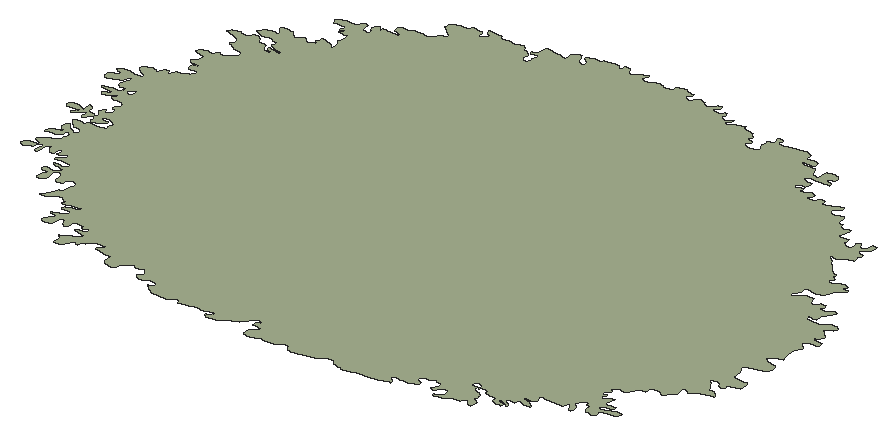
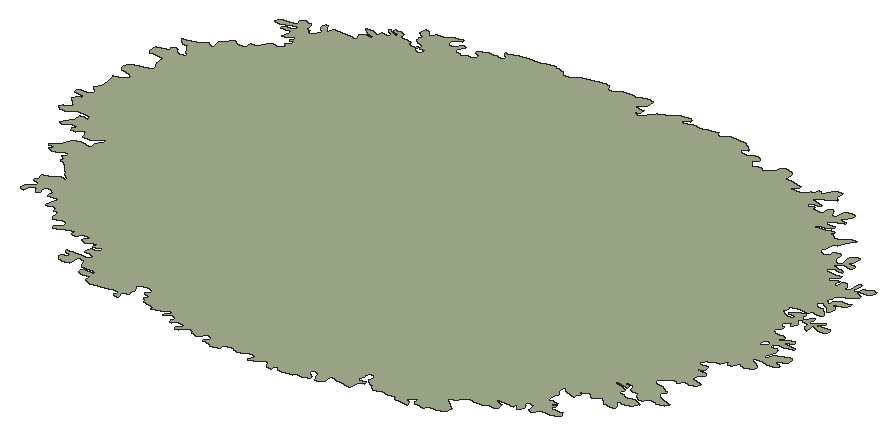
# SketchUp Ruby script. Lengths in inches.
U = 1.inch
M = Sketchup.active_model
def pt(a) = Geom::Point3d.new(a.map { |v| v * U })
def face(e, loops, mat)
  f = e.add_face(loops[0].map { |a| pt(a) })
  loops[1..].each { |l| e.add_face(l.map { |a| pt(a) }).erase! }
  f.material = f.back_material = mat if mat
  f
end
# faces: each face lists its corners as indices into pts; further lists are holes
def faces(e, pts, list, mat = nil) = list.each { |f| face(e, (f[0].is_a?(Array) ? f : [f]).map { |l| l.map { |i| pts[i] } }, mat) }
# xy, xz, yz: faces in a plane at the given z, y or x. An outline is a flat list of corners, or four numbers for a rectangle; further outlines are holes
def ring(l) = l.size == 4 ? [[l[0], l[1]], [l[2], l[1]], [l[2], l[3]], [l[0], l[3]]] : l.each_slice(2).to_a
def flat(e, list, mat, &to3) = list.each { |f| face(e, (f[0].is_a?(Array) ? f : [f]).map { |l| ring(l).map { |u, v| to3.(u, v) } }, mat) }
def xy(e, z, list, mat = nil) = flat(e, list, mat) { |x, y| [x, y, z] }
def xz(e, y, list, mat = nil) = flat(e, list, mat) { |x, z| [x, y, z] }
def yz(e, x, list, mat = nil) = flat(e, list, mat) { |y, z| [x, y, z] }
def lines(e, pts, list) = list.each { |a, b| e.add_line(pt(pts[a]), pt(pts[b])) }
# prism: a flat outline (further loops are holes) pulled along v
def prism(e, loops, v, mat = nil)
  f = face(e, loops, mat); d = Geom::Vector3d.new(v.map { |x| x * U })
  f.pushpull(f.normal.samedirection?(d) ? d.length : -d.length)
end
def box(e, o, s, mat = nil) = prism(e, [[o, [o[0] + s[0], o[1], o[2]], [o[0] + s[0], o[1] + s[1], o[2]], [o[0], o[1] + s[1], o[2]]]], [0, 0, s[2]], mat)
def at(x, y, z, deg = 0) = Geom::Transformation.translation(pt([x, y, z])) * Geom::Transformation.rotation(ORIGIN, Z_AXIS, deg.degrees)
def axes(o, x, y, z) = Geom::Transformation.new([*x, 0, *y, 0, *z, 0, *pt(o).to_a, 1])
def part(name) = M.definitions.add(name)
# library, detail: a bought-in or finely detailed component or shape, given as its bounding box
def library(name, o, s) = part(name).tap { |d| box(d.entities, o, s) }
def detail(e, o, s) = box(e.add_group.entities, o, s)
def put(e, d, t, mat = nil) = e.add_instance(d, t).tap { |i| i.material = mat if mat }
def group(e, t, mat = nil) = e.add_group.tap { |g| g.transformation = t; g.material = mat if mat }.entities
root = M.entities
M.materials.add("Boxwoodplan").color = [166, 177, 144]
xy(root,9.058,[[[182.292,67.129,182.181,67.133,182.086,67.159,182.03,67.215,182.028,67.317,182.054,67.382,182.118,67.445,182.167,67.509,182.225,67.606,182.039,67.635,181.949,67.644,181.969,67.732,182.055,67.79,182.086,67.8,182.081,67.846,181.992,67.877,181.876,67.837,181.779,67.706,181.636,67.551,181.475,67.464,181.37,67.441,181.309,67.416,181.293,67.373,181.149,67.281,180.955,67.251,180.866,67.26,180.786,67.306,180.786,67.328,180.831,67.359,180.922,67.437,180.99,67.483,180.901,67.498,180.788,67.48,180.668,67.436,180.572,67.445,180.475,67.454,180.378,67.447,180.251,67.403,180.051,67.356,179.962,67.349,179.924,67.443,179.916,67.465,179.849,67.473,179.76,67.454,179.591,67.336,179.391,67.328,179.161,67.353,178.994,67.446,178.853,67.61,179.036,67.702,178.936,67.756,178.8,67.772,178.674,67.749,178.602,67.697,178.521,67.672,178.405,67.738,178.363,67.806,178.451,67.847,178.477,67.907,178.482,67.957,178.441,68.009,178.369,68.085,178.283,68.117,178.196,68.064,178.13,68.038,178.074,68.08,178.057,68.103,178.033,68.121,178.004,68.111,177.924,68.058,177.853,68.01,177.777,67.923,177.765,67.79,177.694,67.749,177.644,67.723,177.584,67.725,177.485,67.746,177.398,67.793,177.354,67.861,177.346,67.951,177.355,68.018,177.368,68.04,177.349,68.08,177.135,68.1,177.203,68.135,177.177,68.136,177.084,68.13,176.914,68.146,176.837,68.173,176.82,68.206,176.835,68.224,176.96,68.314,176.958,68.371,176.873,68.393,176.714,68.39,176.583,68.319,176.486,68.233,176.411,68.199,176.364,68.172,176.363,68.154,176.399,68.101,176.383,68.046,176.313,68.081,176.249,68.121,176.188,68.072,176.166,68.017,176.134,67.904,176.087,67.855,176.014,67.822,175.923,67.816,175.853,67.841,175.834,67.874,175.841,67.892,175.862,67.932,175.884,67.991,175.853,68.048,175.752,68.149,175.866,68.229,175.927,68.269,176.007,68.285,176.074,68.315,176.129,68.37,176.214,68.476,176.142,68.503,176.0625,68.511,175.93,68.53,175.892,68.565,175.899,68.584,175.974,68.62,176.136,68.657,176.178,68.709,176.173,68.748,176.147,68.764,175.997,68.711,175.951,68.732,175.952,68.752,175.975,68.814,175.814,68.825,175.733,68.833,175.679,68.826,175.672,68.806,175.656,68.71,175.641,68.642,175.599,68.591,175.552,68.578,175.533,68.594,175.474,68.639,175.429,68.757,175.39,68.783,175.363,68.784,175.309,68.777,175.302,68.757,175.3,68.641,175.246,68.523,175.185,68.449,175.105,68.419,175.026,68.422,174.98,68.448,174.947,68.506,174.947,68.564,175.001,68.677,175.115,68.784,175.135,68.803,175.122,68.823,175.095,68.829,175.015,68.847,174.934,68.86,174.907,68.875,174.914,68.895,174.934,68.914,175.083,68.982,175.245,69.005,175.287,69.108,175.26,69.169,175.213,69.191,175.186,69.187,175.023,69.168,174.982,69.2,174.989,69.22,175.016,69.279,175.174,69.334,175.346,69.403,175.394,69.442,175.381,69.463,175.284,69.436,175.113,69.417,174.969,69.372,174.88,69.386,174.853,69.392,174.859,69.412,174.88,69.426,174.935,69.47,174.907,69.507,174.88,69.503,174.797,69.511,174.742,69.56,174.728,69.601,174.701,69.597,174.618,69.575,174.461,69.489,174.312,69.413,174.238,69.38,174.183,69.392,174.196,69.412,174.215,69.452,174.242,69.469,174.266,69.55,174.316,69.65,174.348,69.759,174.399,69.812,174.472,69.852,174.516,69.972,174.538,70.112,174.558,70.227,174.554,70.285,174.509,70.321,174.428,70.335,174.342,70.335,174.268,70.31,174.258,70.245,174.259,70.184,174.226,70.124,174.138,70.087,174.081,70.096,174.043,70.155,174.032,70.216,174.006,70.337,174.001,70.4,173.96,70.453,173.933,70.475,173.895,70.491,173.836,70.479,173.802,70.46,173.8,70.428,173.792,70.366,173.795,70.229,173.82,70.167,173.812,70.103,173.761,70.038,173.713,70.01,173.675,69.998,173.637,70.003,173.595,70.011,173.577,70.039,173.573,70.166,173.594,70.223,173.639,70.276,173.655,70.306,173.647,70.334,173.59,70.34,173.508,70.346,173.471,70.362,173.448,70.39,173.445,70.453,173.46,70.483,173.495,70.499,173.667,70.472,173.746,70.497,173.795,70.526,173.856,70.573,173.869,70.636,173.846,70.662,173.802,70.664,173.725,70.67,173.633,70.681,173.532,70.717,173.513,70.746,173.519,70.76,173.538,70.763,173.598,70.775,173.773,70.761,173.863,70.787,173.875,70.844,173.849,70.907,173.777,70.946,173.698,70.953,173.585,70.946,173.485,70.921,173.402,70.939,173.398,70.968,173.418,70.997,173.465,71.054,173.531,71.11,173.584,71.19,173.576,71.224,173.531,71.241,173.466,71.24,173.348,71.14,173.308,71.141,173.274,71.161,173.296,71.22,173.312,71.287,173.269,71.35,173.229,71.366,173.209,71.367,173.203,71.352,173.207,71.306,173.204,71.164,173.163,71.102,173.124,71.108,173.089,71.131,172.991,71.262,172.967,71.327,172.942,71.355,172.927,71.344,172.871,71.293,172.836,71.234,172.856,71.103,172.861,71.037,172.841,70.971,172.791,70.962,172.757,70.978,172.747,71.023,172.767,71.155,172.776,71.233,172.776,71.27,172.761,71.282,172.746,71.272,172.667,71.237,172.627,71.183,172.618,71.12,172.579,71.077,172.442,70.987,172.402,70.977,172.358,70.986,172.278,71.026,172.258,71.056,172.262,71.089,172.295,71.151,172.392,71.237,172.482,71.263,172.572,71.263,172.667,71.267,172.606,71.318,172.455,71.404,172.438,71.466,172.491,71.503,172.583,71.573,172.702,71.635,172.82,71.709,172.856,71.723,172.882,71.746,172.908,71.789,172.911,71.882,172.944,72.003,172.945,72.065,172.924,72.086,172.902,72.095,172.839,72.109,172.806,72.104,172.802,72.088,172.814,71.996,172.772,71.934,172.724,71.899,172.647,71.871,172.576,71.858,172.415,71.833,172.38,71.839,172.367,71.853,172.367,71.86,172.376,71.901,172.393,71.947,172.435,71.995,172.504,72.042,172.563,72.063,172.621,72.065,172.66,72.068,172.68,72.075,172.703,72.096,172.698,72.121,172.644,72.151,172.576,72.207,172.544,72.264,172.54,72.331,172.553,72.382,172.605,72.426,172.631,72.432,172.642,72.425,172.662,72.411,172.705,72.35,172.754,72.304,172.882,72.226,172.956,72.192,172.991,72.177,173.011,72.184,173.035,72.206,173.042,72.222,173.053,72.263,173.038,72.32,172.995,72.366,172.963,72.389,172.929,72.401,172.869,72.401,172.795,72.404,172.752,72.446,172.666,72.519,172.607,72.569,172.568,72.617,172.569,72.646,172.593,72.671,172.649,72.698,172.684,72.703,172.725,72.7,172.785,72.679,172.847,72.677,172.883,72.684,172.917,72.726,172.966,72.757,173.025,72.764,173.096,72.764,173.25,72.771,173.39,72.792,173.423,72.808,173.424,72.826,173.418,72.868,173.406,72.913,173.417,72.957,173.447,73.06,173.434,73.083,173.411,73.097,173.354,73.126,173.301,73.164,173.228,73.192,173.155,73.195,173.105,73.184,173.084,73.17,173.059,73.119,173.064,73.098,173.075,73.093,173.099,73.088,173.25,73.076,173.276,73.071,173.281,73.0625,173.272,73.046,173.232,73.007,173.187,72.964,173.122,72.928,173.06,72.884,172.988,72.849,172.951,72.852,172.931,72.863,172.906,72.9,172.899,72.995,172.882,73.02,172.9,73.034,172.906,73.077,172.9,73.088,172.889,73.088,172.874,73.087,172.848,73.083,172.816,73.076,172.798,73.065,172.717,72.97,172.685,72.915,172.654,72.892,172.631,72.895,172.605,72.916,172.596,72.932,172.59,72.973,172.619,73.057,172.624,73.102,172.615,73.13,172.595,73.137,172.557,73.128,172.537,73.114,172.491,73.064,172.369,72.957,172.333,72.932,172.307,72.927,172.27,72.935,172.258,72.951,172.349,73.057,172.412,73.102,172.426,73.129,172.425,73.145,172.416,73.152,172.405,73.148,172.39,73.143,172.359,73.131,172.275,73.108,172.108,73.089,172.035,73.096,171.987,73.121,171.965,73.149,171.964,73.165,171.981,73.217,172.029,73.264,172.089,73.281,172.16,73.284,172.234,73.266,172.362,73.223,172.448,73.197,172.459,73.201,172.459,73.22,172.45,73.239,172.425,73.287,172.424,73.342,172.431,73.407,172.443,73.437,172.46,73.45,172.509,73.413,172.548,73.363,172.575,73.317,172.585,73.255,172.597,73.204,172.612,73.176,172.635,73.175,172.77,73.157,172.843,73.144,172.878,73.14,172.896,73.154,172.911,73.202,172.856,73.244,172.797,73.309,172.78,73.335,172.78,73.352,172.814,73.46,172.844,73.483,172.871,73.489,172.886,73.477,172.895,73.459,172.924,73.414,172.935,73.39,172.947,73.391,172.968,73.404,173.048,73.482,173.065,73.528,173.066,73.579,173.052,73.611,173.031,73.623,172.968,73.646,172.928,73.666,172.92,73.687,172.936,73.736,172.992,73.773,173.026,73.795,173.039,73.816,173.047,73.869,173.045,73.916,172.95,73.992,172.806,74.014,172.744,74.031,172.709,74.013,172.681,74.014,172.612,74.031,172.593,74.058,172.602,74.082,172.728,74.185,172.722,74.217,172.7,74.233,172.655,74.225,172.626,74.216,172.5,74.154,172.46,74.107,172.411,74.063,172.342,74.049,172.314,74.05,172.267,74.102,172.295,74.126,172.3125,74.165,172.344,74.188,172.438,74.22,172.483,74.25,172.472,74.281,172.459,74.283,172.449,74.276,172.423,74.27,172.384,74.273,172.249,74.284,172.102,74.3125,172.078,74.327,172.084,74.347,172.109,74.375,172.322,74.435,172.385,74.434,172.446,74.419,172.506,74.391,172.533,74.393,172.539,74.403,172.588,74.48,172.612,74.495,172.618,74.515,172.618,74.583,172.607,74.593,172.594,74.591,172.536,74.591,172.479,74.585,172.432,74.568,172.408,74.576,172.387,74.596,172.362,74.63,172.342,74.718,172.353,74.806,172.383,74.848,172.389,74.88,172.402,74.923,172.439,74.944,172.435,74.99,172.413,75.026,172.324,75.003,172.306,74.969,172.307,74.95,172.31,74.886,172.23,74.839,172.089,74.745,171.933,74.7,171.849,74.725,171.807,74.778,171.798,74.904,171.926,74.99,172.009,75.003,172.052,75.027,172.076,75.061,172.075,75.081,171.989,75.112,171.916,75.138,171.854,75.194,171.889,75.249,171.965,75.278,172.061,75.312,172.126,75.311,172.305,75.267,172.397,75.246,172.482,75.25,172.533,75.269,172.539,75.289,172.523,75.355,172.462,75.407,172.417,75.415,172.305,75.485,172.258,75.527,172.244,75.564,172.237,75.617,172.237,75.644,172.25,75.659,172.292,75.695,172.343,75.709,172.457,75.741,172.488,75.751,172.528,75.75,172.578,75.746,172.591,75.733,172.606,75.703,172.62,75.689,172.63,75.689,172.658,75.692,172.674,75.704,172.695,75.754,172.723,75.787,172.739,75.81,172.742,75.835,172.758,75.86,172.778,75.872,172.826,75.884,172.865,75.877,172.886,75.833,172.89,75.781,172.907,75.755,172.928,75.754,172.97,75.796,172.995,75.838,173.009,75.942,173.025,75.968,173.057,75.975,173.089,75.974,173.108,75.963,173.129,75.94,173.161,75.94,173.214,75.961,173.258,76.007,173.272,76.032,173.261,76.046,173.321,76.043,173.35,76.046,173.366,76.066,173.371,76.114,173.405,76.155,173.439,76.2,173.385,76.243,173.318,76.272,173.281,76.271,173.248,76.261,173.206,76.249,173.164,76.255,173.142,76.271,173.121,76.295,173.098,76.397,173.111,76.423,173.116,76.439,173.126,76.443,173.231,76.463,173.277,76.472,173.295,76.483,173.285,76.486,173.199,76.514,173.133,76.526,173.105,76.519,173.07,76.52,173.034,76.52,172.998,76.532,172.96,76.582,172.942,76.611,172.942,76.642,172.957,76.663,172.986,76.678,173.017,76.697,173.025,76.725,173.055,76.782,173.082,76.836,173.088,76.89,173.081,76.917,173.041,76.928,172.963,76.954,172.79,77.001,172.754,77.018,172.737,77.042,172.773,77.097,172.817,77.131,172.863,77.159,172.918,77.178,172.97,77.1875,173.023,77.184,173.078,77.16,173.133,77.162,173.16,77.167,173.173,77.187,173.19,77.228,173.227,77.264,173.248,77.282,173.274,77.284,173.343,77.267,173.405,77.256,173.431,77.253,173.455,77.268,173.542,77.336,173.629,77.401,173.683,77.498,173.679,77.542,173.638,77.579,173.521,77.617,173.395,77.647,173.309,77.719,173.251,77.755,173.182,77.776,173.155,77.788,173.141,77.808,173.163,77.855,173.211,77.896,173.209,77.981,173.159,78.06,173.029,78.116,172.741,78.212,172.72,78.246,172.792,78.31,172.913,78.362,173.018,78.367,173.075,78.353,173.119,78.327,173.168,78.317,173.221,78.326,173.282,78.337,173.311,78.368,173.326,78.448,173.343,78.483,173.397,78.482,173.454,78.471,173.502,78.451,173.569,78.392,173.593,78.358,173.607,78.318,173.608,78.249,173.614,78.245,173.623,78.249,173.65,78.262,173.701,78.268,173.79,78.271,173.87,78.235,173.904,78.17,173.929,78.092,173.999,78.047,174.039,78.035,174.057,78.034,174.084,78.043,174.179,78.05,174.196,78.055,174.176,78.071,174.113,78.095,174.061,78.099,174.023,78.118,174.004,78.152,174.001,78.164,174.004,78.184,174.019,78.191,174.054,78.192,174.096,78.185,174.202,78.156,174.317,78.152,174.369,78.159,174.387,78.162,174.413,78.173,174.369,78.203,174.328,78.213,174.242,78.228,174.184,78.242,174.143,78.244,174.121,78.248,174.096,78.263,174.044,78.289,173.997,78.315,173.975,78.348,173.985,78.404,174.014,78.442,174.055,78.471,174.015,78.502,173.96,78.517,173.917,78.52,173.862,78.528,173.831,78.555,173.813,78.591,173.799,78.6,173.77,78.599,173.654,78.571,173.602,78.557,173.553,78.559,173.505,78.562,173.456,78.578,173.408,78.595,173.368,78.602,173.282,78.65,173.307,78.662,173.309,78.669,173.32,78.709,173.336,78.745,173.362,78.782,173.393,78.814,173.437,78.839,173.49,78.862,173.535,78.873,173.641,78.867,173.718,78.862,173.751,78.858,173.762,78.857,173.762,78.87,173.754,78.912,173.733,78.956,173.697,78.995,173.654,79.026,173.621,79.073,173.623,79.096,173.634,79.117,173.681,79.147,173.733,79.17,173.76,79.169,173.786,79.163,173.84,79.148,173.908,79.142,173.955,79.127,173.979,79.114,173.997,79.095,174.041,79.055,174.08,79.02,174.125,78.989,174.181,78.976,174.235,78.981,174.28,79.01,174.312,79.046,174.361,79.084,174.387,79.083,174.409,79.069,174.45,79.027,174.497,78.994,174.625,79.019,174.699,79.037,174.74,79.065,174.746,79.085,174.725,79.102,174.674,79.124,174.664,79.147,174.672,79.169,174.688,79.214,174.695,79.273,174.699,79.299,174.722,79.315,174.749,79.316,174.779,79.308,174.821,79.288,174.955,79.248,175.016,79.226,175.055,79.193,175.082,79.153,175.097,79.13,175.104,79.123,175.113,79.126,175.121,79.131,175.154,79.176,175.16,79.212,175.15,79.315,175.128,79.362,175.104,79.397,175.069,79.436,175.059,79.466,175.07,79.477,175.081,79.475,175.103,79.476,175.102,79.484,175.107,79.508,175.1,79.549,175.085,79.705,175.087,79.782,174.972,79.802,174.875,79.804,174.8125,79.8125,174.795,79.819,174.781,79.83,174.794,79.839,174.907,79.882,174.941,79.911,174.94,79.924,174.917,79.948,174.881,79.952,174.828,79.94,174.78,79.918,174.763,79.919,174.748,79.945,174.774,80.028,174.777,80.069,174.776,80.082,174.752,80.103,174.663,80.085,174.55,80.088,174.441,80.105,174.38,80.185,174.378,80.213,174.416,80.25,174.512,80.303,174.561,80.33,174.615,80.335,174.74,80.332,174.831,80.337,174.891,80.346,174.931,80.384,174.971,80.418,174.979,80.461,175.005,80.5,175.061,80.513,175.098,80.509,175.141,80.475,175.152,80.389,175.159,80.3,175.183,80.257,175.238,80.231,175.33,80.212,175.385,80.234,175.403,80.276,175.38,80.319,175.333,80.355,175.277,80.442,175.313,80.521,175.387,80.603,175.406,80.606,175.43,80.576,175.449,80.528,175.523,80.447,175.551,80.421,175.542,80.475,175.524,80.57,175.58,80.587,175.641,80.582,175.768,80.578,175.881,80.575,176.003,80.557,176.021,80.557,176.009,80.587,175.958,80.629,175.828,80.681,175.79,80.689,175.767,80.735,175.769,80.826,175.804,80.871,175.853,80.896,175.969,80.901,176.066,80.91,176.161,80.977,176.287,80.982,176.403,80.971,176.499,80.953,176.62,80.946,176.663,80.991,176.676,81.038,176.719,81.133,176.808,81.187,176.928,81.244,176.94,81.26,176.923,81.294,176.882,81.332,176.775,81.413,176.707,81.487,176.649,81.528,176.592,81.57,176.623,81.577,176.622,81.591,176.617,81.612,176.606,81.679,176.609,81.709,176.644,81.744,176.727,81.785,176.81,81.821,176.848,81.827,176.904,81.826,176.991,81.816,177.014,81.808,177.038,81.81,177.07,81.843,177.122,81.918,177.158,81.932,177.215,81.936,177.317,81.93,177.413,81.898,177.445,81.877,177.474,81.835,177.475,81.765,177.478,81.736,177.483,81.715,177.506,81.704,177.559,81.715,177.604,81.745,177.666,81.798,177.691,81.822,177.712,81.834,177.725,81.85,177.64,81.897,177.602,81.913,177.559,81.956,177.534,82.036,177.535,82.067,177.593,82.083,177.785,82.055,177.882,82.039,177.917,82.026,177.917,81.98,177.927,81.952,177.987,81.948,178.091,81.962,178.193,81.975,178.235,81.971,178.282,81.957,178.309,81.934,178.334,81.933,178.359,81.943,178.503,81.972,178.544,81.981,178.596,81.987,178.632,81.984,178.677,81.957,178.707,81.886,178.733,81.863,178.778,81.844,178.818,81.833,178.858,81.808,178.91,81.753,178.964,81.696,178.951,81.619,178.944,81.545,178.958,81.515,178.989,81.485,179.016,81.461,179.063,81.453,179.099,81.45,179.144,81.481,179.157,81.512,179.158,81.553,179.146,81.628,179.183,81.787,179.172,81.817,179.154,81.829,179.13,81.833,179.091,81.834,179.039,81.828,179.003,81.826,178.956,81.835,178.931,81.858,178.938,81.88,178.966,81.896,179.005,81.91,179.05,81.937,179.075,82.013,179.079,82.178,179.079,82.21,179.102,82.228,179.128,82.233,179.227,82.222,179.426,82.201,179.517,82.19,179.606,82.169,179.693,82.153,179.744,82.147,179.739,82.355,179.807,82.427,179.892,82.486,179.946,82.477,179.974,82.441,180.022,82.37,180.045,82.297,180.053,82.26,180.051,82.241,180.078,82.206,180.183,82.173,180.235,82.173,180.274,82.204,180.277,82.279,180.174,82.36,180.096,82.419,180.108,82.453,180.152,82.49,180.246,82.541,180.296,82.55,180.377,82.538,180.481,82.537,180.504,82.615,180.714,82.643,180.814,82.661,180.922,82.647,181.001,82.578,181.034,82.543,181.061,82.541,181.101,82.568,181.099,82.643,181.09,82.685,181.103,82.72,181.153,82.729,181.208,82.715,181.279,82.621,181.3,82.548,181.333,82.513,181.382,82.498,181.433,82.503,181.479,82.53,181.567,82.613,181.648,82.668,181.75,82.715,181.798,82.7,181.812,82.663,181.76,82.592,181.734,82.557,181.742,82.515,181.831,82.457,181.931,82.443,181.981,82.452,182.031,82.498,182.109,82.566,182.224,82.581,182.339,82.553,182.37,82.523,182.447,82.492,182.547,82.511,182.629,82.565,182.629,82.678,182.686,82.721,182.799,82.745,182.904,82.74,182.985,82.681,183.131,82.66,183.185,82.651,183.191,82.614,183.117,82.546,183.084,82.473,183.096,82.437,183.168,82.396,183.27,82.401,183.323,82.433,183.343,82.472,183.363,82.544,183.412,82.567,183.436,82.579,183.487,82.579,183.59,82.541,183.633,82.47,183.719,82.417,183.849,82.447,183.884,82.478,183.89,82.52,183.93,82.603,184.037,82.622,184.067,82.592,184.073,82.55,184.02,82.466,183.972,82.448,183.945,82.413,184.005,82.349,184.136,82.337,184.227,82.373,184.294,82.444,184.319,82.45,184.328,82.433,184.346,82.392,184.37,82.357,184.359,82.301,184.339,82.257,184.357,82.222,184.446,82.179,184.554,82.184,184.609,82.203,184.66,82.258,184.677,82.273,184.679,82.255,184.666,82.212,184.593,82.132,184.559,82.102,184.57,82.066,184.617,82.047,184.675,82.048,184.771,82.088,184.853,82.146,185.073,82.225,185.095,82.153,185.118,82.123,185.169,82.118,185.285,82.11,185.409,82.084,185.424,82.013,185.447,81.983,185.493,81.964,185.516,81.93,185.502,81.892,185.475,81.795,185.592,81.773,185.638,81.755,185.648,81.72,185.574,81.65,185.56,81.613,185.576,81.579,185.652,81.527,185.755,81.5,185.856,81.496,185.968,81.563,186.01,81.639,185.952,81.71,185.919,81.779,185.939,81.885,185.948,81.922,185.919,81.956,185.915,81.992,185.957,82.018,186.058,82.022,186.047,82.122,186.005,82.274,186.055,82.287,186.12,82.275,186.173,82.256,186.204,82.199,186.154,82.131,186.158,82.095,186.204,82.076,186.312,82.076,186.442,82.111,186.949,82.178,186.995,82.168,187.041,82.145,187.087,82.121,187.121,82.097,187.152,82.027,187.135,81.935,187.339,81.949,187.404,81.943,187.489,81.911,187.526,81.805,187.511,81.757,187.495,81.724,187.454,81.717,187.284,81.749,187.22,81.755,187.177,81.755,187.157,81.749,187.154,81.733,187.182,81.685,187.223,81.666,187.27,81.666,187.443,81.681,187.512,81.683,187.596,81.648,187.633,81.609,187.664,81.546,187.732,81.437,187.811,81.398,187.896,81.394,187.927,81.435,187.921,81.518,187.903,81.571,187.91,81.637,187.951,81.687,188.052,81.719,188.161,81.732,188.25,81.701,188.298,81.659,188.332,81.597,188.333,81.551,188.271,81.495,188.205,81.482,188.164,81.471,188.132,81.437,188.136,81.407,188.185,81.389,188.283,81.363,188.354,81.339,188.374,81.306,188.362,81.275,188.308,81.247,188.221,81.24,188.059,81.233,187.972,81.222,187.883,81.256,187.819,81.269,187.737,81.251,187.681,81.208,187.679,81.143,187.737,81.103,187.824,81.081,187.91,81.066,187.957,81.066,187.991,81.046,188.012,81.003,187.995,80.938,187.96,80.89,187.932,80.866,187.887,80.854,187.745,80.834,187.725,80.829,187.716,80.784,187.72,80.751,187.765,80.732,187.832,80.731,187.873,80.731,187.923,80.746,187.986,80.778,188,80.712,187.971,80.665,187.964,80.635,188.003,80.617,188.064,80.622,188.146,80.67,188.202,80.711,188.23,80.736,188.268,80.721,188.332,80.704,188.401,80.651,188.397,80.603,188.354,80.537,188.321,80.472,188.339,80.448,188.386,80.445,188.462,80.456,188.544,80.495,188.583,80.554,188.655,80.597,188.715,80.609,188.752,80.601,188.77,80.577,188.773,80.548,188.756,80.521,188.728,80.497,188.73,80.483,188.751,80.481,188.923,80.499,189.004,80.51,189.071,80.552,189.113,80.589,189.192,80.614,189.289,80.619,189.312,80.595,189.315,80.566,189.155,80.349,189.17,80.304,189.227,80.251,189.31,80.237,189.399,80.255,189.467,80.283,189.552,80.305,189.617,80.213,189.653,79.999,189.655,79.985,189.691,79.974,189.775,79.996,189.786,79.918,189.81,79.871,189.886,79.861,190.023,79.896,190.091,79.893,190.106,79.839,190.038,79.619,190.027,79.567,190.05,79.514,190.116,79.486,190.184,79.496,190.32,79.523,190.34,79.419,190.335,79.316,190.457,79.247,190.59,79.216,190.62,79.318,190.61,79.421,190.587,79.474,190.615,79.525,190.684,79.535,190.723,79.482,190.745,79.429,190.793,79.395,190.87,79.418,190.924,79.467,190.948,79.583,190.952,79.636,191.013,79.659,191.07,79.631,191.1,79.577,191.075,79.455,190.96,79.375,190.907,79.339,190.886,79.282,190.866,79.231,190.889,79.186,191.021,79.161,191.077,79.134,191.082,79.083,191.009,78.997,191.044,78.895,191.073,78.844,191.061,78.794,190.927,78.768,190.826,78.729,190.722,78.658,190.671,78.623,190.605,78.626,190.541,78.659,190.509,78.667,190.483,78.643,190.527,78.549,190.646,78.483,190.693,78.445,190.69,78.396,190.775,78.32,190.941,78.132,191.073,78.05,191.136,78.035,191.173,77.992,191.158,77.898,191.274,77.834,191.211,77.749,191.191,77.697,191.189,77.673,191.22,77.661,191.357,77.679,191.492,77.755,191.622,77.768,191.747,77.734,191.75,77.687,191.684,77.66,191.658,77.644,191.672,77.62,191.75,77.599,191.822,77.596,191.854,77.595,191.867,77.571,191.779,77.482,191.613,77.322,191.589,77.232,191.585,77.187,191.557,77.142,191.464,77.067,191.336,77.038,191.211,77.043,191.102,77.082,191.033,77.076,191.006,77.004,191.033,76.894,191.004,76.787,190.886,76.72,190.914,76.62,191.052,76.642,191.224,76.833,191.451,76.815,191.527,76.605,191.572,76.595,191.654,76.618,191.741,76.723,191.879,76.735,191.917,76.635,191.867,76.574,191.852,76.539,191.929,76.501,192.068,76.531,192.1875,76.598,192.234,76.614,192.324,76.592,192.302,76.477,192.191,76.384,192.126,76.289,192.134,76.113,192.12,76.078,192.027,76.056,191.895,76.087,191.92,75.981,192.051,75.941,192.197,75.936,192.346,75.965,192.583,76.087,192.719,76.099,192.811,76.008,192.778,75.905,192.638,75.849,192.591,75.825,192.5625,75.766,192.666,75.675,192.817,75.515,192.784,75.414,192.668,75.359,192.632,75.335,192.67,75.274,192.814,75.269,192.944,75.247,192.956,75.145,192.883,75.089,192.75,75.078,192.625,75.041,192.582,74.942,192.75,74.761,192.643,74.568,192.646,74.388,192.7,74.176,192.744,74.078,192.612,74.051,192.489,74.008,192.395,73.931,192.368,73.869,192.479,73.801,192.731,73.744,192.808,73.662,192.829,73.559,192.787,73.467,192.672,73.394,192.211,73.234,192.213,73.141,192.257,73.048,192.311,72.954,192.3125,72.863,192.307,72.803,192.304,72.773,192.33,72.719,192.451,72.676,192.576,72.672,192.702,72.682,192.744,72.68,192.802,72.633,192.813,72.453,192.786,72.395,192.677,72.347,192.55,72.33,192.509,72.331,192.463,72.281,192.505,72.191,192.492,72.163,192.407,72.144,192.366,72.145,192.296,72.17,192.264,72.26,192.194,72.292,192.071,72.297,192.029,72.291,192.013,72.233,192.089,72.156,192.176,71.992,192.204,71.969,192.23,71.918,192.248,71.888,192.329,71.877,192.409,71.86,192.494,71.792,192.557,71.71,192.554,71.681,192.47,71.656,192.221,71.616,192.026,71.488,191.953,71.469,191.858,71.544,191.818,71.553,191.754,71.52,191.757,71.435,191.813,71.27,191.771,71.264,191.738,71.219,191.689,71.18,191.635,71.066,191.596,71.019,191.562,71,191.526,71.013,191.404,71.1,191.341,71.115,191.298,71.116,191.253,71.098,191.19,71.063,191.16,70.991,191.17,70.938,191.152,70.874,190.99,70.852,190.938,70.81,190.906,70.759,190.859,70.718,190.847,70.655,190.816,70.609,190.782,70.583,190.745,70.573,190.676,70.564,190.578,70.575,190.518,70.55,190.456,70.502,190.426,70.457,190.501,70.419,190.528,70.376,190.492,70.32,190.437,70.284,190.416,70.225,190.415,70.209,190.414,70.194,190.433,70.186,190.505,70.18,190.531,70.182,190.551,70.182,190.555,70.166,190.517,70.097,190.498,70.049,190.495,70.02,190.536,70.018,190.675,70.094,190.744,70.11,190.825,70.107,190.809,70.004,190.791,69.89,190.791,69.843,190.814,69.82,190.854,69.818,190.918,69.845,190.999,69.846,191.058,69.832,191.098,69.827,191.104,69.798,191.064,69.76,190.985,69.73,190.919,69.722,190.836,69.696,190.797,69.658,190.78,69.602,190.784,69.587,190.824,69.586,190.906,69.611,191.064,69.673,191.218,69.703,191.344,69.705,191.396,69.685,191.371,69.611,191.35,69.569,191.289,69.518,191.136,69.492,190.997,69.491,190.936,69.482,190.905,69.427,190.931,69.308,190.916,69.264,190.835,69.243,190.699,69.255,190.641,69.261,190.597,69.314,190.588,69.426,190.588,69.468,190.576,69.496,190.567,69.511,190.547,69.512,190.489,69.525,190.484,69.581,190.486,69.595,190.482,69.61,190.463,69.614,190.383,69.617,190.326,69.591,190.281,69.536,190.244,69.499,190.219,69.44,190.23,69.391,190.286,69.354,190.361,69.254,190.357,69.155,190.348,69.115,190.341,69.088,190.31,69.066,190.29,69.067,190.269,69.098,190.24,69.157,190.175,69.258,190.134,69.298,190.12,69.312,190.109,69.299,190.102,69.271,190.099,69.227,190.08,69.173,190.074,69.16,190.044,69.144,189.961,69.137,189.82,69.139,189.534,69.14,189.476,69.162,189.389,69.173,189.37,69.163,189.364,69.133,189.414,69.074,189.439,68.976,189.433,68.936,189.401,68.896,189.377,68.889,189.317,68.88,189.214,68.88,189.116,68.884,189.068,68.853,189.123,68.829,189.224,68.814,189.332,68.78,189.407,68.726,189.488,68.654,189.47,68.629,189.409,68.614,189.308,68.621,189.271,68.63,189.22,68.65,189.172,68.684,189.122,68.708,189.087,68.63,189.077,68.558,189.037,68.545,188.981,68.558,188.936,68.589,188.923,68.6,188.905,68.608,188.893,68.59,188.859,68.513,188.861,68.485,188.894,68.448,188.986,68.416,189.025,68.383,189.038,68.34,189.036,68.326,189.017,68.323,188.974,68.36,188.894,68.409,188.801,68.427,188.744,68.429,188.732,68.415,188.753,68.39,188.867,68.347,188.904,68.335,188.927,68.292,188.923,68.264,188.922,68.251,188.879,68.249,188.766,68.26,188.661,68.295,188.626,68.325,188.617,68.371,188.616,68.441,188.565,68.461,188.506,68.442,188.406,68.449,188.307,68.467,188.28,68.489,188.255,68.526,188.259,68.568,188.265,68.583,188.227,68.591,188.133,68.616,188.076,68.619,188.041,68.606,188.029,68.577,188.009,68.571,187.982,68.597,187.979,68.612,188.009,68.635,188.025,68.646,188.017,68.671,187.93,68.729,187.893,68.752,187.874,68.756,187.833,68.736,187.793,68.716,187.773,68.71,187.762,68.681,187.785,68.59,187.88,68.587,187.919,68.582,187.949,68.541,187.942,68.513,187.936,68.499,187.944,68.471,188.055,68.434,188.143,68.396,188.204,68.338,188.221,68.3125,188.22,68.299,188.185,68.283,188.165,68.273,188.196,68.251,188.251,68.225,188.263,68.2,188.212,68.168,188.2,68.141,188.225,68.106,188.31,68.062,188.388,67.994,188.387,67.851,188.366,67.825,188.314,67.814,188.26,67.829,188.222,67.874,188.182,67.939,188.164,67.949,188.126,67.944,188.074,67.926,188.052,67.897,188.053,67.854,188.052,67.84,188.019,67.828,187.842,67.819,187.834,67.826,187.786,67.808,187.742,67.777,187.658,67.692,187.606,67.661,187.532,67.651,187.394,67.643,187.34,67.658,187.338,67.698,187.447,67.762,187.547,67.834,187.544,67.937,187.538,67.98,187.538,67.994,187.507,68.015,187.447,68.034,187.373,68.034,187.289,67.95,187.269,67.911,187.212,67.866,187.197,67.857,187.161,67.865,187.124,67.88,187.112,67.907,187.152,67.999,187.212,68.094,187.213,68.135,187.145,68.189,187.034,68.224,186.982,68.246,186.945,68.238,186.92,68.215,186.886,68.171,186.853,68.156,186.811,68.157,186.755,68.166,186.718,68.168,186.68,68.145,186.599,68.05,186.613,68.01,186.687,67.97,186.742,67.938,186.769,67.917,186.778,67.89,186.754,67.851,186.694,67.807,186.592,67.756,186.537,67.735,186.464,67.738,186.409,67.76,186.335,67.769,186.29,67.745,186.253,67.743,186.221,67.76,186.166,67.766,186.093,67.752,186.071,67.717,186.081,67.659,186.178,67.575,186.205,67.536,186.206,67.51,186.206,67.497,186.188,67.492,185.898,67.391,185.623,67.369,185.39,67.373,185.299,67.371,185.177,67.31,185.074,67.275,184.977,67.279,184.939,67.281,184.89,67.299,184.842,67.328,184.781,67.325,184.692,67.334,184.608,67.376,184.548,67.433,184.517,67.478,184.458,67.491,184.359,67.479,184.263,67.438,184.183,67.398,184.084,67.325,183.987,67.269,183.894,67.24,183.653,67.222,183.463,67.186,183.366,67.19,183.301,67.284,183.27,67.351,183.182,67.365,183.091,67.352,182.995,67.28,182.93,67.217,182.84,67.21,182.663,67.233,182.478,67.24,182.4,67.189],[172.8,74.415,172.842,74.419,172.862,74.422,172.888,74.431,172.9,74.474,172.901,74.513,172.908,74.597,172.9,74.631,172.888,74.643,172.888,74.658,172.845,74.635,172.789,74.612,172.769,74.606,172.753,74.59,172.732,74.557,172.722,74.52,172.724,74.476,172.743,74.437,172.762,74.421]]],"Boxwoodplan")
